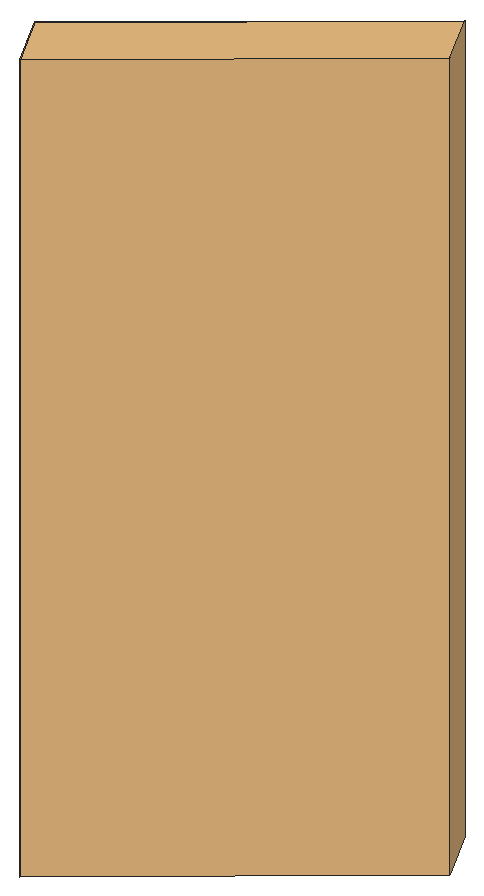
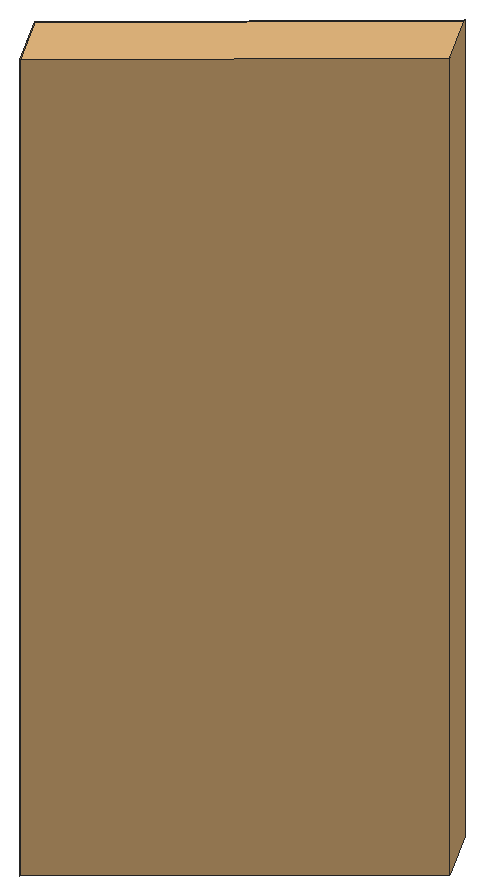
# SketchUp Ruby script. Lengths in inches.
U = 1.inch
M = Sketchup.active_model
def pt(a) = Geom::Point3d.new(a.map { |v| v * U })
def face(e, loops, mat)
  f = e.add_face(loops[0].map { |a| pt(a) })
  loops[1..].each { |l| e.add_face(l.map { |a| pt(a) }).erase! }
  f.material = f.back_material = mat if mat
  f
end
# faces: each face lists its corners as indices into pts; further lists are holes
def faces(e, pts, list, mat = nil) = list.each { |f| face(e, (f[0].is_a?(Array) ? f : [f]).map { |l| l.map { |i| pts[i] } }, mat) }
# xy, xz, yz: faces in a plane at the given z, y or x. An outline is a flat list of corners, or four numbers for a rectangle; further outlines are holes
def ring(l) = l.size == 4 ? [[l[0], l[1]], [l[2], l[1]], [l[2], l[3]], [l[0], l[3]]] : l.each_slice(2).to_a
def flat(e, list, mat, &to3) = list.each { |f| face(e, (f[0].is_a?(Array) ? f : [f]).map { |l| ring(l).map { |u, v| to3.(u, v) } }, mat) }
def xy(e, z, list, mat = nil) = flat(e, list, mat) { |x, y| [x, y, z] }
def xz(e, y, list, mat = nil) = flat(e, list, mat) { |x, z| [x, y, z] }
def yz(e, x, list, mat = nil) = flat(e, list, mat) { |y, z| [x, y, z] }
def lines(e, pts, list) = list.each { |a, b| e.add_line(pt(pts[a]), pt(pts[b])) }
# prism: a flat outline (further loops are holes) pulled along v
def prism(e, loops, v, mat = nil)
  f = face(e, loops, mat); d = Geom::Vector3d.new(v.map { |x| x * U })
  f.pushpull(f.normal.samedirection?(d) ? d.length : -d.length)
end
def box(e, o, s, mat = nil) = prism(e, [[o, [o[0] + s[0], o[1], o[2]], [o[0] + s[0], o[1] + s[1], o[2]], [o[0], o[1] + s[1], o[2]]]], [0, 0, s[2]], mat)
def at(x, y, z, deg = 0) = Geom::Transformation.translation(pt([x, y, z])) * Geom::Transformation.rotation(ORIGIN, Z_AXIS, deg.degrees)
def axes(o, x, y, z) = Geom::Transformation.new([*x, 0, *y, 0, *z, 0, *pt(o).to_a, 1])
def part(name) = M.definitions.add(name)
# library, detail: a bought-in or finely detailed component or shape, given as its bounding box
def library(name, o, s) = part(name).tap { |d| box(d.entities, o, s) }
def detail(e, o, s) = box(e.add_group.entities, o, s)
def put(e, d, t, mat = nil) = e.add_instance(d, t).tap { |i| i.material = mat if mat }
def group(e, t, mat = nil) = e.add_group.tap { |g| g.transformation = t; g.material = mat if mat }.entities
root = M.entities
c1 = library("sm2 st v2 Component\#1",[0,0,0],[29.46,4.93,43.46])
put(root,c1,axes([64.08,86.58,49.21],[0.3444,0.28084,0],[-0.22623,0.42754,0],[0,0,0.6557]))
